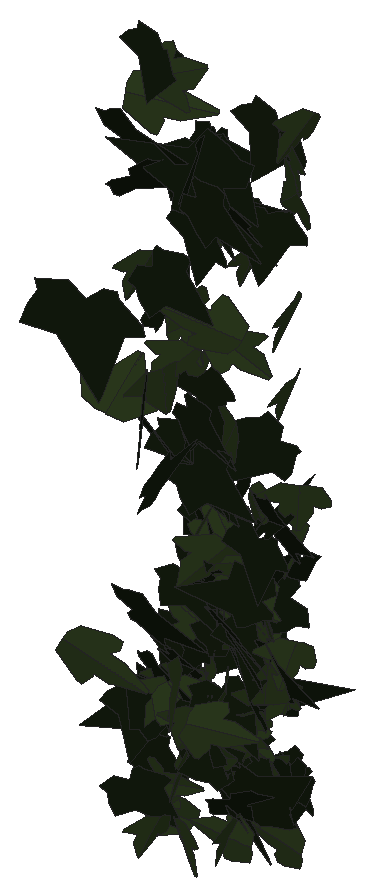
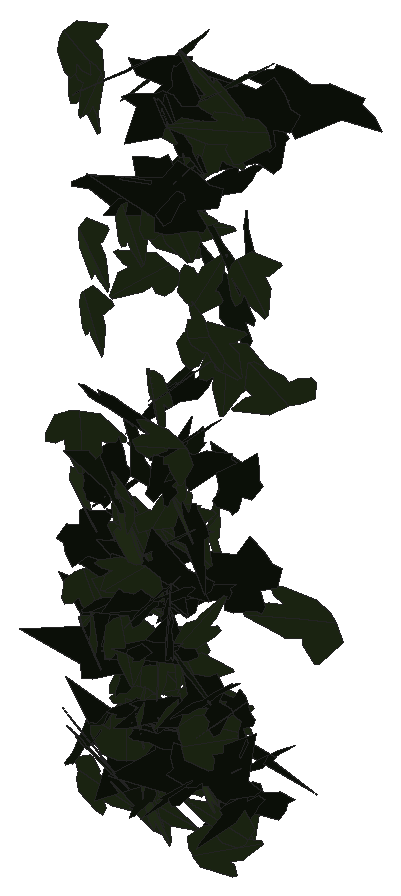
# SketchUp Ruby script. Lengths in inches.
U = 1.inch
M = Sketchup.active_model
def pt(a) = Geom::Point3d.new(a.map { |v| v * U })
def face(e, loops, mat)
  f = e.add_face(loops[0].map { |a| pt(a) })
  loops[1..].each { |l| e.add_face(l.map { |a| pt(a) }).erase! }
  f.material = f.back_material = mat if mat
  f
end
# faces: each face lists its corners as indices into pts; further lists are holes
def faces(e, pts, list, mat = nil) = list.each { |f| face(e, (f[0].is_a?(Array) ? f : [f]).map { |l| l.map { |i| pts[i] } }, mat) }
# xy, xz, yz: faces in a plane at the given z, y or x. An outline is a flat list of corners, or four numbers for a rectangle; further outlines are holes
def ring(l) = l.size == 4 ? [[l[0], l[1]], [l[2], l[1]], [l[2], l[3]], [l[0], l[3]]] : l.each_slice(2).to_a
def flat(e, list, mat, &to3) = list.each { |f| face(e, (f[0].is_a?(Array) ? f : [f]).map { |l| ring(l).map { |u, v| to3.(u, v) } }, mat) }
def xy(e, z, list, mat = nil) = flat(e, list, mat) { |x, y| [x, y, z] }
def xz(e, y, list, mat = nil) = flat(e, list, mat) { |x, z| [x, y, z] }
def yz(e, x, list, mat = nil) = flat(e, list, mat) { |y, z| [x, y, z] }
def lines(e, pts, list) = list.each { |a, b| e.add_line(pt(pts[a]), pt(pts[b])) }
# prism: a flat outline (further loops are holes) pulled along v
def prism(e, loops, v, mat = nil)
  f = face(e, loops, mat); d = Geom::Vector3d.new(v.map { |x| x * U })
  f.pushpull(f.normal.samedirection?(d) ? d.length : -d.length)
end
def box(e, o, s, mat = nil) = prism(e, [[o, [o[0] + s[0], o[1], o[2]], [o[0] + s[0], o[1] + s[1], o[2]], [o[0], o[1] + s[1], o[2]]]], [0, 0, s[2]], mat)
def at(x, y, z, deg = 0) = Geom::Transformation.translation(pt([x, y, z])) * Geom::Transformation.rotation(ORIGIN, Z_AXIS, deg.degrees)
def axes(o, x, y, z) = Geom::Transformation.new([*x, 0, *y, 0, *z, 0, *pt(o).to_a, 1])
def part(name) = M.definitions.add(name)
# library, detail: a bought-in or finely detailed component or shape, given as its bounding box
def library(name, o, s) = part(name).tap { |d| box(d.entities, o, s) }
def detail(e, o, s) = box(e.add_group.entities, o, s)
def put(e, d, t, mat = nil) = e.add_instance(d, t).tap { |i| i.material = mat if mat }
def group(e, t, mat = nil) = e.add_group.tap { |g| g.transformation = t; g.material = mat if mat }.entities
root = M.entities
M.materials.add("1026 AP 7946 SUNNY SIDE UP").color = [254, 231, 186]
M.materials.add("efeu1").color = [18, 25, 13]
M.materials.add("efeu2").color = [43, 57, 29]
c1 = part("ivyleaf_9")
p = [[1.54,2.16,1.25],[1.36,2.04,1.19],[-0.21,0.99,0.68],[-0.71,1.11,0.82],[-0.85,0.86,0.67],[-0.8,0.17,0.21],
  [-0.9,-0.01,0.1],[-0.67,-0.16,-0.02],[-0.08,-0.08,-0.05],[-0.03,-0.6,-0.4],[0.65,-0.88,-0.66],[0.83,-0.6,-0.49],
  [1.29,-0.42,-0.43],[1.8125,-0.07,-0.26],[1.21,0.44,0.15]]
faces(c1.entities,p,[[0,1,2,3,4,5,6,7,8,9,10,11,12,13,14]],"efeu1")
c2 = part("ivyleaf_10")
p = [[0,0.5,-0.03],[-0.0625,2.02,-0.43],[-0.19,2.01,-0.46],[-0.54,1.05,-0.29],[-0.52,0.625,-0.18],[-0.83,0.76,-0.28],
  [-1.16,0.64,-0.33],[-1.15,0.33,-0.24],[-0.77,-0.39,0.02],[-0.3,-0.51,0.16],[0.04,-0.48,0.23],[-0.02,2.01,-0.4375],
  [-0.06,2.01,-0.43],[0.04,-0.49,0.23],[0.67,-0.49,0.14],[1.38,0.36,-0.2],[1.375,0.51,-0.24],[0.81,0.65,-0.19],
  [0.62,0.59,-0.15],[0.6,1.09,-0.28],[0.5,1.23,-0.31]]
faces(c2.entities,p,[[0,1,2,3,4,5,6,7,8,9,10],[11,12,0,13,14,15,16,17,18,19,20]],"efeu2")
put(root,c1,axes([117.83,208.5,277.38],[-0.42484,-0.22091,-0.2723],[0.34773,0.14426,-0.35794],[0.41334,-0.34842,0.02124]),"1026 AP 7946 SUNNY SIDE UP")
put(root,c2,axes([118.54,209.6,271.15],[0.07238,-0.10882,0.38652],[0.34776,-0.3049,-0.12065],[0.50747,0.22447,0.02755]),"1026 AP 7946 SUNNY SIDE UP")
put(root,c1,axes([118.3,209.31,274.1875],[0.014,0.34013,0.19518],[-0.00989,-0.18743,0.34943],[0.61065,-0.01083,0.00118]),"1026 AP 7946 SUNNY SIDE UP")
put(root,c1,axes([117.9,209.72,275.49],[-0.11193,-0.00481,-0.39147],[0.51084,-0.20129,-0.06125],[-0.30993,-0.33004,0.04042]),"1026 AP 7946 SUNNY SIDE UP")
put(root,c2,axes([116.48,210.1,270.73],[-0.24251,0.00215,-0.36169],[0.53948,-0.08057,-0.15624],[-0.11732,-0.37493,0.02921]),"1026 AP 7946 SUNNY SIDE UP")
put(root,c1,axes([118.46,210.22,278.47],[0.32959,-0.21648,-0.20712],[-0.11867,0.1976,-0.30093],[0.44778,0.21171,0.07271]),"1026 AP 7946 SUNNY SIDE UP")
put(root,c2,axes([117.93,210.5,268.19],[-0.25309,0.19162,-0.13327],[0.10207,-0.11521,-0.25752],[-0.34992,-0.1722,0.02128]),"1026 AP 7946 SUNNY SIDE UP")
put(root,c1,axes([117.58,210.36,277],[0.19487,-0.19916,-0.27591],[-0.09052,0.26746,-0.23176],[0.51548,0.12226,0.0636]),"1026 AP 7946 SUNNY SIDE UP")
put(root,c1,axes([117,210.64,271.27],[0.24588,-0.12273,0.27151],[0.31106,-0.17544,-0.20558],[0.33633,0.25199,-0.00836]),"1026 AP 7946 SUNNY SIDE UP")
put(root,c2,axes([117.35,210.625,268.04],[-0.1028,-0.26277,0.06989],[-0.0142,-0.06917,-0.27925],[0.42709,-0.06555,0.00754]),"1026 AP 7946 SUNNY SIDE UP")
put(root,c2,axes([118.25,210.5,269.96],[-0.0716,-0.13412,-0.31858],[0.38368,0.2011,-0.126],[0.36406,-0.23831,0.07014]),"1026 AP 7946 SUNNY SIDE UP")
put(root,c2,axes([118.4375,210.81,276.11],[0.13383,0.09713,0.33186],[-0.40162,-0.19676,0.12971],[0.34309,-0.26822,0.0224]),"1026 AP 7946 SUNNY SIDE UP")
put(root,c2,axes([117.96,210.8125,269.85],[-0.28019,-0.19913,0.09285],[-0.07422,-0.07997,-0.27519],[0.33634,-0.18354,0.01662]),"1026 AP 7946 SUNNY SIDE UP")
put(root,c1,axes([118.08,210.64,273.92],[0.18134,-0.1899,-0.27722],[-0.093,0.26741,-0.21985],[0.50806,0.11673,0.05871]),"1026 AP 7946 SUNNY SIDE UP")
put(root,c1,axes([118.25,210.9,278.32],[-0.24324,0.07737,0.3766],[-0.57389,0.05131,-0.1702],[-0.12276,-0.39321,0.04946]),"1026 AP 7946 SUNNY SIDE UP")
put(root,c1,axes([116.79,210.83,268.4],[0.01502,-0.13794,-0.24831],[0.09328,0.23584,-0.13568],[0.4255,-0.04683,0.03851]),"1026 AP 7946 SUNNY SIDE UP")
put(root,c1,axes([116.46,211.04,278.4],[0.13081,-0.08906,0.32278],[0.33984,-0.22754,-0.12688],[0.38421,0.23158,0.00233]),"1026 AP 7946 SUNNY SIDE UP")
put(root,c1,axes([116.92,210.7,278.11],[0.31941,0.25236,0.1837],[0.19628,0.12632,-0.33261],[-0.44305,0.2379,-0.01492]),"1026 AP 7946 SUNNY SIDE UP")
put(root,c2,axes([116.42,210.83,274.33],[0.36029,0.20232,-0.20601],[0.20563,0.15477,0.31478],[0.39867,-0.26267,0.02381]),"1026 AP 7946 SUNNY SIDE UP")
put(root,c1,axes([118.79,211.12,271.85],[-0.29715,0.0334,0.21825],[-0.33357,-0.06893,-0.18432],[0.04748,-0.27525,0.07091]),"1026 AP 7946 SUNNY SIDE UP")
put(root,c1,axes([117.68,210.98,274.53],[0.26164,-0.21139,-0.14057],[-0.09124,0.12547,-0.27484],[0.3839,0.17389,0.03048]),"1026 AP 7946 SUNNY SIDE UP")
put(root,c1,axes([117.45,210.77,276.19],[-0.04475,0.21769,0.34596],[-0.09325,0.3294,-0.22407],[-0.62069,-0.06518,0.00872]),"1026 AP 7946 SUNNY SIDE UP")
put(root,c1,axes([117.6,211.33,277.2],[-0.04785,-0.27243,0.17846],[0.01278,-0.17614,-0.28241],[0.50879,-0.0212,0.02388]),"1026 AP 7946 SUNNY SIDE UP")
put(root,c1,axes([117.8,211.33,278.625],[-0.07586,0.00181,-0.33444],[0.31668,-0.25726,-0.03382],[-0.40039,-0.20382,0.03662]),"1026 AP 7946 SUNNY SIDE UP")
put(root,c1,axes([118.15,211.14,270.18],[-0.03189,-0.25293,-0.19859],[0.02702,0.19057,-0.26029],[0.49795,-0.02654,0.0014]),"1026 AP 7946 SUNNY SIDE UP")
put(root,c2,axes([117.09,211.11,274.82],[-0.20134,-0.32249,-0.08272],[0.06454,0.06807,-0.35682],[0.51787,-0.13386,0.01231]),"1026 AP 7946 SUNNY SIDE UP")
put(root,c1,axes([118.68,211.15,268.57],[-0.15303,0.06975,0.30787],[0.39328,-0.16292,0.1223],[0.27855,0.26834,-0.00353]),"1026 AP 7946 SUNNY SIDE UP")
put(root,c2,axes([117.84,211.25,268.98],[-0.25909,0.0509,0.247],[0.35753,-0.07519,0.1772],[0.1427,0.28079,0.00449]),"1026 AP 7946 SUNNY SIDE UP")
put(root,c2,axes([118.24,211.26,268.09],[0.11864,-0.33227,0.05377],[0.0103,-0.05396,-0.35129],[0.52924,0.07553,-0.00522]),"1026 AP 7946 SUNNY SIDE UP")
put(root,c1,axes([117.59,211.16,273.54],[0.19062,-0.23173,-0.14769],[-0.03751,0.14587,-0.26527],[0.42574,0.11661,0.04276]),"1026 AP 7946 SUNNY SIDE UP")
put(root,c2,axes([118.44,211.16,267.89],[0.00308,0.04167,0.31171],[-0.47964,-0.0095,0.00333],[0.0155,-0.30219,0.04108]),"1026 AP 7946 SUNNY SIDE UP")
put(root,c1,axes([118.1875,211.18,269.03],[-0.39266,-0.11145,-0.11902],[-0.18238,-0.02075,0.28031],[-0.17346,0.2741,-0.02529]),"1026 AP 7946 SUNNY SIDE UP")
put(root,c1,axes([117.99,211.2,271.26],[0.38654,-0.13863,-0.0029],[-0.01725,-0.01534,-0.29019],[0.21733,0.24536,-0.01788]),"1026 AP 7946 SUNNY SIDE UP")
put(root,c1,axes([118.41,211.04,268.58],[0.38117,0.18494,0.05954],[0.08883,0.01933,-0.31342],[-0.29092,0.24822,-0.01768]),"1026 AP 7946 SUNNY SIDE UP")
put(root,c2,axes([117.9,211.37,272.22],[-0.24338,-0.22667,0.22482],[-0.13967,-0.20331,-0.28199],[0.47609,-0.17552,0.0322]),"1026 AP 7946 SUNNY SIDE UP")
put(root,c2,axes([117.6875,211.4,270.19],[-0.08901,0.09052,-0.29727],[0.12017,-0.28029,-0.10748],[-0.46089,-0.09056,0.02939]),"1026 AP 7946 SUNNY SIDE UP")
put(root,c2,axes([117.32,211.36,275.12],[-0.25739,-0.17123,0.18791],[-0.14598,-0.16208,-0.24223],[0.3665,-0.18481,0.03549]),"1026 AP 7946 SUNNY SIDE UP")
put(root,c1,axes([118.24,211.43,270.78],[0.0872,-0.19924,0.19599],[0.08928,-0.18281,-0.21408],[0.42513,0.07926,0.00476]),"1026 AP 7946 SUNNY SIDE UP")
put(root,c1,axes([118.54,211.44,272.57],[-0.05358,-0.30176,0.07604],[-0.00789,-0.07544,-0.31327],[0.48907,-0.03428,0.00327]),"1026 AP 7946 SUNNY SIDE UP")
put(root,c1,axes([116.8,211.32,269.4],[-0.47057,0.07074,0.0646],[-0.10639,-0.01682,-0.31525],[-0.1032,-0.30522,0.03046]),"1026 AP 7946 SUNNY SIDE UP")
put(root,c1,axes([116.43,211.45,269.24],[-0.10835,-0.27814,0.08416],[-0.00767,-0.08447,-0.2953],[0.45647,-0.06744,0.01501]),"1026 AP 7946 SUNNY SIDE UP")
put(root,c2,axes([118.78,211.31,270.24],[-0.28533,-0.21604,-0.02856],[-0.0392,-0.01364,0.29039],[-0.34,0.18288,-0.00951]),"1026 AP 7946 SUNNY SIDE UP")
put(root,c2,axes([117.28,211.4,268.77],[0.20782,-0.26291,0.14839],[0.0962,-0.13211,-0.30389],[0.46261,0.14558,-0.00347]),"1026 AP 7946 SUNNY SIDE UP")
put(root,c2,axes([118.24,211.12,275.71],[0.23632,0.14315,0.23045],[0.19673,0.18752,-0.20989],[-0.36714,0.19262,0.03587]),"1026 AP 7946 SUNNY SIDE UP")
put(root,c2,axes([117.33,211.45,275.81],[-0.10196,-0.18799,-0.23417],[-0.15274,-0.20499,0.20296],[-0.43658,0.11562,-0.01632]),"1026 AP 7946 SUNNY SIDE UP")
put(root,c2,axes([118.4,211.26,269.75],[-0.27943,-0.23707,-0.03713],[0.05145,0.01878,-0.30474],[0.37321,-0.18009,0.01421]),"1026 AP 7946 SUNNY SIDE UP")
put(root,c2,axes([118.15,211.14,270.19],[0.05275,-0.23661,-0.21731],[-0.01811,0.20972,-0.24457],[0.4967,0.03278,0.01416]),"1026 AP 7946 SUNNY SIDE UP")
put(root,c2,axes([117.29,211.18,269.81],[0.22761,0.27432,0.14984],[0.1246,0.12075,-0.31857],[-0.47087,0.16456,-0.01187]),"1026 AP 7946 SUNNY SIDE UP")
put(root,c2,axes([116.59,211.39,276.37],[-0.07724,-0.30028,0.1021],[-0.00516,-0.10153,-0.31379],[0.49803,-0.04762,0.01258]),"1026 AP 7946 SUNNY SIDE UP")
put(root,c2,axes([117.12,211.48,269.68],[-0.22243,-0.21656,0.21001],[-0.06961,-0.20922,-0.26028],[0.46379,-0.13526,0.06165]),"1026 AP 7946 SUNNY SIDE UP")
put(root,c2,axes([117.16,211.39,269.21],[-0.20993,0.02864,0.27511],[0.40736,-0.06426,0.14024],[0.11045,0.29142,0.00569]),"1026 AP 7946 SUNNY SIDE UP")
put(root,c1,axes([117.38,211.42,277.84],[0.26777,-0.29732,-0.02205],[-0.03047,0.01161,-0.35273],[0.46755,0.17104,-0.01036]),"1026 AP 7946 SUNNY SIDE UP")
put(root,c2,axes([117.17,211.45,267.7],[-0.13792,-0.05189,-0.26372],[-0.37829,-0.08832,0.10296],[-0.15877,0.25549,-0.01623]),"1026 AP 7946 SUNNY SIDE UP")
put(root,c1,axes([118.63,211.53,270.55],[0.1622,-0.1368,0.30689],[0.234,-0.25962,-0.17698],[0.46051,0.18011,-0.01816]),"1026 AP 7946 SUNNY SIDE UP")
put(root,c1,axes([118.23,211.33,269.41],[0.00988,-0.20181,-0.20185],[0.0356,0.19457,-0.20578],[0.4396,-0.01122,0.0212]),"1026 AP 7946 SUNNY SIDE UP")
put(root,c1,axes([118.05,211.46,268.33],[0.25587,-0.25044,0.02654],[0.00236,-0.03139,-0.30744],[0.3961,0.16197,-0.01531]),"1026 AP 7946 SUNNY SIDE UP")
put(root,c2,axes([118.3125,211.29,269.43],[-0.22022,-0.15265,-0.19664],[0.25746,0.10341,-0.20931],[0.28389,-0.21219,0.03728]),"1026 AP 7946 SUNNY SIDE UP")
put(root,c2,axes([119.1,211.48,271.01],[-0.25731,-0.22077,0.08939],[0.02127,-0.11535,-0.2728],[0.37311,-0.14567,0.0772]),"1026 AP 7946 SUNNY SIDE UP")
put(root,c2,axes([118.93,211.57,270.18],[-0.11372,-0.02597,-0.27892],[-0.2885,-0.20195,0.0693],[-0.3154,0.19409,0.03717]),"1026 AP 7946 SUNNY SIDE UP")
put(root,c1,axes([118.48,211.58,271.02],[-0.20265,-0.29937,0.0094],[0.01644,-0.01627,-0.33546],[0.47075,-0.1283,0.01576]),"1026 AP 7946 SUNNY SIDE UP")
put(root,c2,axes([119.22,211.33,268],[0.02814,0.02738,0.32475],[-0.4932,0.04189,0.01485],[-0.06359,-0.31279,0.02854]),"1026 AP 7946 SUNNY SIDE UP")
put(root,c2,axes([118.43,211.45,271.96],[0.38519,-0.02441,-0.21304],[-0.32678,-0.01216,-0.25237],[0.01696,0.32027,-0.02393]),"1026 AP 7946 SUNNY SIDE UP")
put(root,c2,axes([117.68,211.46,269.6875],[0.02157,0.25289,-0.11825],[-0.01779,-0.11576,-0.26154],[-0.43727,0.01719,0.00481]),"1026 AP 7946 SUNNY SIDE UP")
put(root,c2,axes([118.72,211.32,271.61],[-0.24203,0.27911,0.05897],[-0.07142,0.03838,-0.32743],[-0.44178,-0.15912,0.02062]),"1026 AP 7946 SUNNY SIDE UP")
put(root,c2,axes([117.54,211.5,272.61],[0.2034,-0.27415,0.07024],[0.02503,-0.0695,-0.31232],[0.44409,0.12948,-0.01456]),"1026 AP 7946 SUNNY SIDE UP")
put(root,c1,axes([116.55,211.53,269.78],[0.26384,-0.06514,-0.23607],[0.36875,-0.00157,0.17765],[-0.06262,-0.28371,0.05147]),"1026 AP 7946 SUNNY SIDE UP")
put(root,c2,axes([116.74,211.4,268.13],[-0.15533,-0.0114,0.26279],[0.38866,0.0646,0.10194],[-0.1011,0.26587,-0.01185]),"1026 AP 7946 SUNNY SIDE UP")
put(root,c1,axes([117.63,211.42,278.43],[-0.1355,-0.18805,-0.28937],[0.25861,0.22867,-0.20916],[0.46277,-0.18285,0.03216]),"1026 AP 7946 SUNNY SIDE UP")
put(root,c2,axes([118.24,211.46,271.89],[-0.36365,-0.12784,0.10349],[-0.12688,-0.06284,-0.27216],[0.22275,-0.24449,0.01392]),"1026 AP 7946 SUNNY SIDE UP")
put(root,c2,axes([118.09,211.44,271.71],[-0.23976,-0.0841,-0.22929],[0.37279,-0.03858,-0.15286],[0.02169,-0.26662,0.09269]),"1026 AP 7946 SUNNY SIDE UP")
put(root,c2,axes([117.22,211.42,278.15],[-0.50916,-0.00136,-0.03181],[0.04852,-0.03213,-0.33213],[-0.00267,-0.32368,0.03119]),"1026 AP 7946 SUNNY SIDE UP")
put(root,c2,axes([118.46,211.53,268.83],[-0.20702,-0.27697,-0.06605],[-0.05786,-0.05172,0.31543],[-0.44271,0.13628,-0.01034]),"1026 AP 7946 SUNNY SIDE UP")
put(root,c2,axes([117.35,211.55,270.83],[-0.01751,0.26437,0.1799],[-0.01678,-0.17345,0.27114],[0.49661,0.00346,0.01551]),"1026 AP 7946 SUNNY SIDE UP")
put(root,c2,axes([118.42,211.59,271.09],[-0.19083,0.11556,-0.2313],[0.144,-0.21275,-0.16457],[-0.371,-0.14202,0.0551]),"1026 AP 7946 SUNNY SIDE UP")
put(root,c1,axes([117.43,211.64,273.4],[0.10983,-0.27732,0.13871],[0.06519,-0.12998,-0.29527],[0.48143,0.08087,0.00834]),"1026 AP 7946 SUNNY SIDE UP")
put(root,c2,axes([118.07,211.39,274.22],[0.2951,-0.2083,-0.1544],[-0.06456,0.15749,-0.27975],[0.3972,0.18035,0.06924]),"1026 AP 7946 SUNNY SIDE UP")
put(root,c1,axes([117.64,211.42,269.68],[0.088,-0.22607,-0.2444],[0.13694,0.24105,-0.21523],[0.49524,-0.02648,0.10294]),"1026 AP 7946 SUNNY SIDE UP")
put(root,c1,axes([118.09,211.71,269.5],[-0.0866,-0.14987,0.23583],[-0.08991,-0.22293,-0.16522],[0.42187,-0.07827,0.0132]),"1026 AP 7946 SUNNY SIDE UP")
put(root,c1,axes([117.25,211.53,271.52],[0.00492,-0.26675,-0.15822],[0.07652,0.15058,-0.27021],[0.4767,-0.02142,0.04501]),"1026 AP 7946 SUNNY SIDE UP")
put(root,c2,axes([119.29,211.35,278.33],[-0.26895,0.13683,0.28455],[-0.37533,0.13967,-0.22337],[-0.30494,-0.2926,0.02396]),"1026 AP 7946 SUNNY SIDE UP")
put(root,c1,axes([118.57,211.71,272.73],[0.10478,-0.12388,0.31849],[0.20981,-0.27973,-0.14641],[0.48095,0.14902,-0.00552]),"1026 AP 7946 SUNNY SIDE UP")
put(root,c1,axes([118.51,211.51,269.84],[0.02818,-0.23985,0.20653],[-0.01549,0.20164,0.24892],[-0.49266,-0.02006,0.00399]),"1026 AP 7946 SUNNY SIDE UP")
put(root,c1,axes([116.58,211.41,268.59],[0.13362,-0.10739,-0.24111],[-0.12042,0.2241,-0.13363],[0.38567,0.10718,0.04181]),"1026 AP 7946 SUNNY SIDE UP")
put(root,c1,axes([118.92,211.77,268.77],[0.01027,-0.21516,0.20792],[-0.00466,-0.20314,-0.22284],[0.46516,0.00271,-0.00682]),"1026 AP 7946 SUNNY SIDE UP")
put(root,c1,axes([119.15,211.63,268.93],[-0.35888,0.07564,-0.12258],[0.16925,-0.05401,-0.2475],[-0.14408,-0.25186,0.01459]),"1026 AP 7946 SUNNY SIDE UP")
put(root,c2,axes([118.98,211.59,275.14],[0.05285,-0.3112,-0.01128],[-0.00448,0.00893,-0.3224],[0.48952,0.03368,-0.00173]),"1026 AP 7946 SUNNY SIDE UP")
put(root,c1,axes([117.36,211.73,274.65],[0.04805,-0.30583,0.02723],[-0.00024,-0.02832,-0.31678],[0.48292,0.03041,-0.00286]),"1026 AP 7946 SUNNY SIDE UP")
put(root,c2,axes([118.78,211.73,270.23],[-0.00487,0.04075,0.29187],[0.36157,-0.16798,0.02652],[0.26741,0.22787,-0.03055]),"1026 AP 7946 SUNNY SIDE UP")
put(root,c1,axes([116.36,211.78,273.37],[0.03429,-0.13451,0.27771],[0.16684,-0.25034,-0.13861],[0.44451,0.10434,0.0306]),"1026 AP 7946 SUNNY SIDE UP")
put(root,c1,axes([118.07,211.6,271.89],[0.14661,0.12242,-0.24252],[-0.24942,-0.17523,-0.15916],[-0.33567,0.18367,0.01234]),"1026 AP 7946 SUNNY SIDE UP")
put(root,c2,axes([117.82,211.58,272.39],[0.14262,0.32645,0.04076],[-0.02893,-0.03402,0.34873],[0.51591,-0.09215,0.00828]),"1026 AP 7946 SUNNY SIDE UP")
put(root,c1,axes([118,211.64,271.33],[0.40926,-0.19967,0.03],[0.01499,-0.03716,-0.33729],[0.31719,0.25938,-0.02277]),"1026 AP 7946 SUNNY SIDE UP")
put(root,c2,axes([118.44,211.5,272.27],[0.2812,-0.07174,-0.23065],[-0.22536,0.18912,-0.17959],[0.29227,0.21485,0.08344]),"1026 AP 7946 SUNNY SIDE UP")
put(root,c1,axes([117.37,211.71,270.48],[-0.35231,0.06222,-0.15692],[0.20984,-0.08282,-0.23701],[-0.15222,-0.25817,0.03646]),"1026 AP 7946 SUNNY SIDE UP")
put(root,c2,axes([117.96,211.81,269.45],[0.02222,-0.05217,0.3172],[0.34927,-0.2154,-0.04931],[0.34583,0.22089,0.02942]),"1026 AP 7946 SUNNY SIDE UP")
put(root,c1,axes([117.16,211.72,273.62],[-0.24706,-0.23294,-0.12405],[0.12253,0.09095,-0.28864],[0.3927,-0.17493,0.01201]),"1026 AP 7946 SUNNY SIDE UP")
put(root,c1,axes([117.65,211.46,271.58],[0.41748,0.13783,0.1095],[0.16331,0.02833,-0.30723],[-0.21867,0.28429,-0.0204]),"1026 AP 7946 SUNNY SIDE UP")
put(root,c2,axes([116.92,211.75,275.46],[0.27163,-0.08084,0.28563],[0.39401,-0.11975,-0.19718],[0.22717,0.30435,0.00047]),"1026 AP 7946 SUNNY SIDE UP")
put(root,c1,axes([116.89,211.61,270.06],[0.40673,-0.08695,0.02182],[0.0196,-0.03065,-0.28013],[0.13954,0.25776,-0.02424]),"1026 AP 7946 SUNNY SIDE UP")
put(root,c1,axes([117.58,211.82,273.04],[0.04693,0.08506,0.33665],[-0.26061,-0.28158,0.08959],[0.46176,-0.16756,0.01635]),"1026 AP 7946 SUNNY SIDE UP")
put(root,c1,axes([118.8,211.73,271.64],[-0.13309,-0.11112,-0.29204],[-0.33999,-0.1843,0.14016],[-0.33577,0.23066,-0.02617]),"1026 AP 7946 SUNNY SIDE UP")
put(root,c1,axes([117.46,211.78,278.41],[-0.31805,0.00634,-0.28276],[0.42369,-0.06096,-0.20635],[-0.083,-0.33548,0.03013]),"1026 AP 7946 SUNNY SIDE UP")
put(root,c1,axes([118.59,211.77,274],[-0.5092,0.00794,-0.02782],[0.04106,-0.03307,-0.33224],[-0.0167,-0.32328,0.0314]),"1026 AP 7946 SUNNY SIDE UP")
put(root,c1,axes([118.625,211.51,270.14],[0.1535,0.0437,0.30505],[0.45892,0.054,-0.10711],[-0.10263,0.30683,-0.02271]),"1026 AP 7946 SUNNY SIDE UP")
put(root,c1,axes([117.43,211.875,272.34],[-0.10438,-0.26515,0.1281],[0.01296,-0.13066,-0.27988],[0.46132,-0.05632,0.03685]),"1026 AP 7946 SUNNY SIDE UP")
put(root,c1,axes([117.37,211.5625,272.59],[0.18956,-0.0346,-0.29879],[-0.45291,0.03667,-0.12772],[0.07431,0.31176,-0.01626]),"1026 AP 7946 SUNNY SIDE UP")
put(root,c2,axes([116.96,211.69,269.8],[-0.33291,-0.18093,0.04463],[-0.02973,-0.04592,-0.28625],[0.29141,-0.21139,0.02178]),"1026 AP 7946 SUNNY SIDE UP")
put(root,c2,axes([119.0625,211.68,273.4],[-0.36279,-0.19927,0.00848],[0.0116,-0.02283,-0.31338],[0.31346,-0.22978,0.02141]),"1026 AP 7946 SUNNY SIDE UP")
put(root,c1,axes([117.61,211.83,269.42],[-0.39818,-0.16682,-0.02526],[0.05457,-0.01,-0.31118],[0.25923,-0.25413,0.0267]),"1026 AP 7946 SUNNY SIDE UP")
put(root,c2,axes([118.4,211.74,271.34],[0.31744,-0.01322,-0.23168],[-0.35283,-0.0374,-0.20554],[-0.03001,0.29983,-0.03407]),"1026 AP 7946 SUNNY SIDE UP")
put(root,c1,axes([116.43,211.9375,279.38],[-0.1383,-0.26967,0.15456],[0.00846,-0.15888,-0.28893],[0.48633,-0.07392,0.04898]),"1026 AP 7946 SUNNY SIDE UP")
put(root,c2,axes([117.54,211.76,277.04],[-0.34596,-0.18157,0.10819],[-0.09937,-0.0893,-0.2931],[0.31535,-0.22734,0.02634]),"1026 AP 7946 SUNNY SIDE UP")
put(root,c1,axes([117.59,211.64,271.6],[-0.37267,0.0686,0.17132],[0.22769,-0.08937,0.25066],[0.16687,0.27515,0.04058]),"1026 AP 7946 SUNNY SIDE UP")
put(root,c2,axes([118.84,211.8,276.22],[0.13368,-0.32625,0.07317],[0.01711,-0.07246,-0.34766],[0.52536,0.08538,-0.0073]),"1026 AP 7946 SUNNY SIDE UP")
put(root,c1,axes([117.27,211.74,269.01],[0.44231,-0.13739,0.11203],[0.13656,-0.07099,-0.32195],[0.24016,0.2934,-0.02325]),"1026 AP 7946 SUNNY SIDE UP")
put(root,c1,axes([118.43,212.01,278.81],[-0.1964,-0.27084,0.16494],[-0.02184,-0.16896,-0.3037],[0.49546,-0.11481,0.05199]),"1026 AP 7946 SUNNY SIDE UP")
put(root,c1,axes([117.61,211.76,271.52],[0.18314,-0.27151,-0.11606],[-0.06821,0.10231,-0.30376],[0.45623,0.12429,0.00118]),"1026 AP 7946 SUNNY SIDE UP")
put(root,c1,axes([117.6,211.73,277.42],[0.45108,-0.10353,0.01764],[0.01094,-0.03268,-0.31302],[0.16479,0.28555,-0.02751]),"1026 AP 7946 SUNNY SIDE UP")
put(root,c1,axes([116.84,211.81,268.98],[0.24793,0.02735,0.27187],[-0.41547,0.042,0.15849],[-0.03505,-0.3044,0.04447]),"1026 AP 7946 SUNNY SIDE UP")
put(root,c2,axes([118.97,211.92,279.15],[-0.05012,-0.27121,0.17796],[-0.00418,-0.17491,-0.28192],[0.5069,-0.02826,0.01527]),"1026 AP 7946 SUNNY SIDE UP")
put(root,c1,axes([118.59,211.57,272.72],[-0.2015,0.29641,-0.04603],[-0.01088,0.04749,0.33271],[0.47162,0.12774,-0.01199]),"1026 AP 7946 SUNNY SIDE UP")
put(root,c2,axes([118.92,211.9,272.59],[0.25226,-0.26041,0.08812],[0.04551,-0.08417,-0.315],[0.42932,0.16194,-0.01838]),"1026 AP 7946 SUNNY SIDE UP")
put(root,c2,axes([116.49,211.875,279.04],[0.27579,-0.14895,-0.28094],[0.3827,-0.12728,0.23286],[-0.30187,-0.29744,0.03855]),"1026 AP 7946 SUNNY SIDE UP")
put(root,c1,axes([118.87,211.875,268.9],[-0.37744,0.07274,-0.09326],[0.11869,-0.06147,-0.25626],[-0.13944,-0.24922,0.03432]),"1026 AP 7946 SUNNY SIDE UP")
put(root,c1,axes([118.13,211.55,273.17],[0.04137,0.09708,0.31328],[0.0401,0.30296,-0.10032],[-0.49951,0.03236,0.01789]),"1026 AP 7946 SUNNY SIDE UP")
put(root,c1,axes([117.34,211.99,271.14],[0.07161,-0.10143,-0.28807],[0.42403,-0.104,0.08367],[-0.19536,-0.26292,0.07603]),"1026 AP 7946 SUNNY SIDE UP")
put(root,c2,axes([116.97,211.97,269.59],[-0.08902,0.01351,-0.27757],[-0.29979,-0.19688,0.02994],[-0.30028,0.19256,0.05239]),"1026 AP 7946 SUNNY SIDE UP")
put(root,c2,axes([117.38,211.89,273.73],[-0.25975,0.02527,-0.27828],[0.36158,-0.15508,-0.16064],[-0.22679,-0.27619,0.0626]),"1026 AP 7946 SUNNY SIDE UP")
put(root,c2,axes([118.11,211.87,276.85],[-0.00389,-0.30317,0.0245],[0.00007,-0.0255,-0.31248],[0.47839,-0.00246,0.00025]),"1026 AP 7946 SUNNY SIDE UP")
put(root,c1,axes([117.18,211.72,277.24],[0.17003,0.03923,0.32819],[0.50417,-0.02222,-0.10951],[0.01351,0.33547,-0.04364]),"1026 AP 7946 SUNNY SIDE UP")
put(root,c1,axes([117.15,211.8,268.86],[0.16181,-0.23005,-0.15433],[-0.02103,0.15423,-0.25479],[0.43004,0.0941,0.04561]),"1026 AP 7946 SUNNY SIDE UP")
put(root,c1,axes([117.77,211.77,270.58],[-0.26359,-0.18626,0.16752],[0.17239,0.12152,0.25887],[-0.3497,0.2003,0.00134]),"1026 AP 7946 SUNNY SIDE UP")
put(root,c1,axes([117.99,212.03,270.64],[-0.32167,-0.18656,0.09146],[-0.0764,-0.07951,-0.28455],[0.31649,-0.2088,0.02427]),"1026 AP 7946 SUNNY SIDE UP")
put(root,c1,axes([117.33,212.04,271.3],[0.02015,-0.06436,-0.30245],[0.39904,-0.15446,0.04544],[-0.25216,-0.24957,0.04775]),"1026 AP 7946 SUNNY SIDE UP")
put(root,c1,axes([118.81,211.97,272.12],[-0.09385,0.12225,-0.25399],[0.11185,-0.23758,-0.1401],[-0.41901,-0.0908,0.01949]),"1026 AP 7946 SUNNY SIDE UP")
put(root,c1,axes([116.78,212,270.31],[-0.02179,-0.29527,0.01798],[0.00179,-0.0192,-0.30463],[0.46526,-0.01376,0.00201]),"1026 AP 7946 SUNNY SIDE UP")
put(root,c1,axes([118.26,211.98,277.37],[-0.30819,-0.22642,-0.09796],[0.12291,0.05609,-0.3074],[0.36525,-0.20993,0.02078]),"1026 AP 7946 SUNNY SIDE UP")
put(root,c2,axes([117.96,211.97,272.09],[0.13378,-0.29946,-0.14005],[0.10498,-0.11999,0.31862],[-0.50522,-0.10423,0.02913]),"1026 AP 7946 SUNNY SIDE UP")
put(root,c2,axes([117.98,211.9,271.71],[-0.34846,-0.08324,-0.15242],[0.26371,-0.07415,-0.21694],[0.03698,-0.25566,0.11076]),"1026 AP 7946 SUNNY SIDE UP")
put(root,c1,axes([116.6,212.07,270],[-0.08911,-0.21833,0.15481],[-0.02937,-0.15127,-0.23263],[0.41683,-0.05733,0.01671]),"1026 AP 7946 SUNNY SIDE UP")
put(root,c2,axes([116.26,211.76,278.69],[0.0009,-0.11521,-0.35492],[0.54194,0.10712,-0.03576],[0.17736,-0.32675,0.11106]),"1026 AP 7946 SUNNY SIDE UP")
put(root,c2,axes([118.6875,211.88,278.66],[-0.31187,0.23162,-0.0553],[0.02912,-0.05634,-0.31363],[-0.37319,-0.19796,0.02173]),"1026 AP 7946 SUNNY SIDE UP")
put(root,c2,axes([118.15,211.91,270.79],[-0.12837,-0.32102,-0.01341],[0.00672,0.01046,-0.34118],[0.50504,-0.08174,0.00113]),"1026 AP 7946 SUNNY SIDE UP")
put(root,c2,axes([118,212.05,272.79],[-0.13444,0.06963,-0.26736],[0.18513,-0.23555,-0.10628],[-0.38046,-0.13922,0.04276]),"1026 AP 7946 SUNNY SIDE UP")
